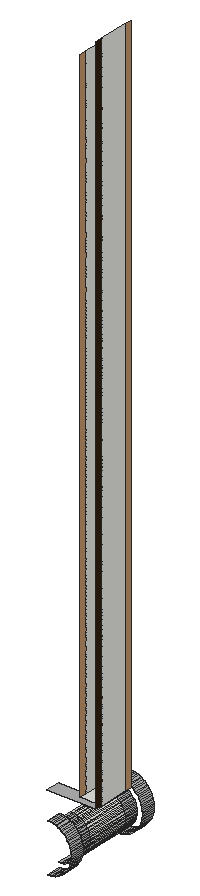
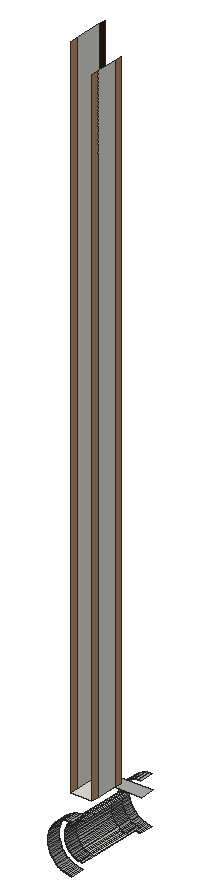
# SketchUp Ruby script. Lengths in inches.
U = 1.inch
M = Sketchup.active_model
def pt(a) = Geom::Point3d.new(a.map { |v| v * U })
def face(e, loops, mat)
  f = e.add_face(loops[0].map { |a| pt(a) })
  loops[1..].each { |l| e.add_face(l.map { |a| pt(a) }).erase! }
  f.material = f.back_material = mat if mat
  f
end
# faces: each face lists its corners as indices into pts; further lists are holes
def faces(e, pts, list, mat = nil) = list.each { |f| face(e, (f[0].is_a?(Array) ? f : [f]).map { |l| l.map { |i| pts[i] } }, mat) }
# xy, xz, yz: faces in a plane at the given z, y or x. An outline is a flat list of corners, or four numbers for a rectangle; further outlines are holes
def ring(l) = l.size == 4 ? [[l[0], l[1]], [l[2], l[1]], [l[2], l[3]], [l[0], l[3]]] : l.each_slice(2).to_a
def flat(e, list, mat, &to3) = list.each { |f| face(e, (f[0].is_a?(Array) ? f : [f]).map { |l| ring(l).map { |u, v| to3.(u, v) } }, mat) }
def xy(e, z, list, mat = nil) = flat(e, list, mat) { |x, y| [x, y, z] }
def xz(e, y, list, mat = nil) = flat(e, list, mat) { |x, z| [x, y, z] }
def yz(e, x, list, mat = nil) = flat(e, list, mat) { |y, z| [x, y, z] }
def lines(e, pts, list) = list.each { |a, b| e.add_line(pt(pts[a]), pt(pts[b])) }
# prism: a flat outline (further loops are holes) pulled along v
def prism(e, loops, v, mat = nil)
  f = face(e, loops, mat); d = Geom::Vector3d.new(v.map { |x| x * U })
  f.pushpull(f.normal.samedirection?(d) ? d.length : -d.length)
end
def box(e, o, s, mat = nil) = prism(e, [[o, [o[0] + s[0], o[1], o[2]], [o[0] + s[0], o[1] + s[1], o[2]], [o[0], o[1] + s[1], o[2]]]], [0, 0, s[2]], mat)
def at(x, y, z, deg = 0) = Geom::Transformation.translation(pt([x, y, z])) * Geom::Transformation.rotation(ORIGIN, Z_AXIS, deg.degrees)
def axes(o, x, y, z) = Geom::Transformation.new([*x, 0, *y, 0, *z, 0, *pt(o).to_a, 1])
def part(name) = M.definitions.add(name)
# library, detail: a bought-in or finely detailed component or shape, given as its bounding box
def library(name, o, s) = part(name).tap { |d| box(d.entities, o, s) }
def detail(e, o, s) = box(e.add_group.entities, o, s)
def put(e, d, t, mat = nil) = e.add_instance(d, t).tap { |i| i.material = mat if mat }
def group(e, t, mat = nil) = e.add_group.tap { |g| g.transformation = t; g.material = mat if mat }.entities
root = M.entities
M.materials.add("Panel-Opening1").color = [191, 148, 107]
M.materials.add("Stained Mahogany").color = [48, 33, 18]
M.materials.add("[Aluminum]").color = [178, 178, 178]
xy(root,65.29,[[211.71,132.28,211.79,133.02]],"[Aluminum]")
xy(root,65.33,[[211.71,127.79,211.79,128.53]],"[Aluminum]")
xy(root,65.58,[[211.71,129.28,211.78,131.53]])
xy(root,65.58,[[211.71,128.53,211.78,129.28],[211.71,131.53,211.78,132.28]],"[Aluminum]")
xy(root,67.55,[[211.71,129.28,211.78,131.53]])
xy(root,67.55,[[211.71,128.53,211.78,129.28],[211.71,131.53,211.78,132.28]],"[Aluminum]")
xy(root,67.8,[[211.71,127.79,211.79,128.53]],"[Aluminum]")
xy(root,67.84,[[211.71,132.28,211.79,133.02]],"[Aluminum]")
xy(root,68.11,[[211.84,129.66,212.96,131.53]])
xy(root,68.11,[[210.46,129.28,210.46,130.03,211.84,130.03,211.84,129.66,212.96,129.66,212.96,129.28]],"[Aluminum]")
yz(root,211.84,[[130.03,68.11,131.15,102.09]])
yz(root,211.84,[[129.66,68.11,130.03,102.09],[131.15,68.11,131.53,102.09]],"Panel-Opening1")
yz(root,212.67,[[129.28,66.4375,131.53,66.5],[129.28,66.5,131.53,66.5625],[129.28,66.5625,131.53,66.63],[129.28,66.63,131.53,66.69]])
yz(root,212.67,[[128.53,66.4375,129.28,66.5],[131.53,66.4375,132.28,66.5],[128.53,66.5,129.28,66.5625],[131.53,66.5,132.28,66.5625],[128.53,66.5625,129.28,66.63],
  [131.53,66.5625,132.28,66.63],[128.53,66.63,129.28,66.69],[131.53,66.63,132.28,66.69]],"[Aluminum]")
yz(root,212.92,[[127.79,66.48,128.53,66.57],[127.79,66.57,128.53,66.65]],"[Aluminum]")
yz(root,212.96,[[129.66,68.11,131.15,103.24]])
yz(root,212.96,[[131.15,68.11,131.53,103.24]],"Panel-Opening1")
yz(root,212.96,[[129.28,68.11,129.66,103.24]],"Stained Mahogany")
yz(root,212.96,[[132.28,66.48,133.02,66.5625],[132.28,66.5625,133.02,66.65]],"[Aluminum]")
p = [[211.79,128.53,65.33],[211.87,128.53,65.34],[211.87,127.79,65.34],[211.79,127.79,65.33],[211.95,128.53,65.35],[211.95,127.79,65.35],
  [211.875,132.28,65.3],[211.79,132.28,65.29],[211.79,133.02,65.29],[211.875,133.02,65.3],[211.96,132.28,65.31],[211.96,133.02,65.31],
  [212.04,132.28,65.33],[212.04,133.02,65.33],[212.11,132.28,65.35],[212.11,133.02,65.35],[212.03,128.53,65.37],[212.03,127.79,65.37],
  [212.1,128.53,65.39],[212.1,127.79,65.39],[212.17,128.53,65.42],[212.17,127.79,65.42],[212.25,128.53,65.46],[212.25,127.79,65.46],
  [212.19,132.28,65.38],[212.19,133.02,65.38],[212.26,132.28,65.42],[212.26,133.02,65.42],[212.34,132.28,65.46],[212.34,133.02,65.46],
  [212.32,128.53,65.5],[212.32,127.79,65.5],[212.38,128.53,65.54],[212.38,127.79,65.54],[212.45,128.53,65.58],[212.45,127.79,65.58],
  [212.41,132.28,65.5],[212.41,133.02,65.5],[212.47,132.28,65.55],[212.47,133.02,65.55],[212.54,132.28,65.6],[212.54,133.02,65.6],
  [212.51,128.53,65.64],[212.51,127.79,65.64],[212.57,128.53,65.69],[212.57,127.79,65.69],[211.84,129.28,65.59],[211.78,129.28,65.58],
  [211.78,128.53,65.58],[211.84,128.53,65.59],[211.9,129.28,65.6],[211.9,128.53,65.6],[211.96,129.28,65.61],[211.96,128.53,65.61],
  [212.02,129.28,65.63],[212.02,128.53,65.63],[212.08,129.28,65.66],[212.08,128.53,65.66],[211.78,131.53,65.58],[211.84,131.53,65.59],
  [211.9,131.53,65.6],[211.96,131.53,65.61],[212.02,131.53,65.63],[212.08,131.53,65.66],[211.78,132.28,65.58],[211.84,132.28,65.59],
  [211.9,132.28,65.6],[211.96,132.28,65.61],[212.02,132.28,65.63],[212.08,132.28,65.66],[212.6,132.28,65.66],[212.6,133.02,65.66],
  [212.62,128.53,65.75],[212.62,127.79,65.75],[212.14,129.28,65.68],[212.14,128.53,65.68],[212.19,129.28,65.71],[212.19,128.53,65.71],
  [212.25,129.28,65.75],[212.25,128.53,65.75],[212.3,129.28,65.78],[212.3,128.53,65.78],[212.14,131.53,65.68],[212.19,131.53,65.71],
  [212.25,131.53,65.75],[212.3,131.53,65.78],[212.14,132.28,65.68],[212.19,132.28,65.71],[212.25,132.28,65.75],[212.3,132.28,65.78],
  [212.65,132.28,65.72],[212.65,133.02,65.72],[212.7,132.28,65.79],[212.7,133.02,65.79],[212.67,128.53,65.8125],[212.67,127.79,65.8125],
  [212.72,128.53,65.88],[212.72,127.79,65.88],[212.35,129.28,65.82],[212.35,128.53,65.82],[212.39,129.28,65.87],[212.39,128.53,65.87],
  [212.35,131.53,65.82],[212.39,131.53,65.87],[212.35,132.28,65.82],[212.39,132.28,65.87],[212.75,132.28,65.85],[212.75,133.02,65.85],
  [212.76,128.53,65.95],[212.76,127.79,65.95],[212.79,128.53,66.02],[212.79,127.79,66.02],[212.44,129.28,65.92],[212.44,128.53,65.92],
  [212.48,129.28,65.97],[212.48,128.53,65.97],[212.44,131.53,65.92],[212.48,131.53,65.97],[212.44,132.28,65.92],[212.48,132.28,65.97],
  [212.79,132.28,65.93],[212.79,133.02,65.93],[212.83,132.28,66],[212.83,133.02,66],[212.83,128.53,66.09],[212.83,127.79,66.09],
  [212.51,129.28,66.02],[212.51,128.53,66.02],[212.55,129.28,66.07],[212.55,128.53,66.07],[212.51,131.53,66.02],[212.55,131.53,66.07],
  [212.51,132.28,66.02],[212.55,132.28,66.07],[212.87,132.28,66.08],[212.87,133.02,66.08],[212.85,128.53,66.17],[212.85,127.79,66.17],
  [212.57,129.28,66.13],[212.57,128.53,66.13],[212.6,129.28,66.1875],[212.6,128.53,66.1875],[212.57,131.53,66.13],[212.6,131.53,66.1875],
  [212.57,132.28,66.13],[212.6,132.28,66.1875],[212.89,132.28,66.15],[212.89,133.02,66.15],[212.875,128.53,66.25],[212.875,127.79,66.25],
  [212.89,128.53,66.32],[212.89,127.79,66.32],[212.625,129.28,66.25],[212.625,128.53,66.25],[212.64,129.28,66.31],[212.64,128.53,66.31],
  [212.625,131.53,66.25],[212.64,131.53,66.31],[212.625,132.28,66.25],[212.64,132.28,66.31],[212.92,132.28,66.23],[212.92,133.02,66.23],
  [212.9375,132.28,66.31],[212.9375,133.02,66.31],[212.91,128.53,66.4],[212.91,127.79,66.4],[212.66,129.28,66.37],[212.66,128.53,66.37],
  [212.66,131.53,66.37],[212.66,132.28,66.37],[212.95,132.28,66.4],[212.95,133.02,66.4],[212.92,128.53,66.48],[212.92,127.79,66.48],
  [212.67,129.28,66.4375],[212.67,128.53,66.4375],[212.67,131.53,66.4375],[212.67,132.28,66.4375],[212.96,132.28,66.48],[212.96,133.02,66.48],
  [212.92,128.53,66.65],[212.91,128.53,66.73],[212.91,127.79,66.73],[212.92,127.79,66.65],[212.95,132.28,66.73],[212.96,132.28,66.65],
  [212.96,133.02,66.65],[212.95,133.02,66.73],[212.89,128.53,66.81],[212.89,127.79,66.81],[212.66,129.28,66.76],[212.67,129.28,66.69],
  [212.67,128.53,66.69],[212.66,128.53,66.76],[212.67,131.53,66.69],[212.66,131.53,66.76],[212.67,132.28,66.69],[212.66,132.28,66.76],
  [212.9375,132.28,66.8125],[212.9375,133.02,66.8125],[212.875,128.53,66.88],[212.875,127.79,66.88],[212.625,129.28,66.88],[212.64,129.28,66.82],
  [212.64,128.53,66.82],[212.625,128.53,66.88],[212.64,131.53,66.82],[212.625,131.53,66.88],[212.64,132.28,66.82],[212.625,132.28,66.88],
  [212.92,132.28,66.9],[212.92,133.02,66.9],[212.85,128.53,66.96],[212.85,127.79,66.96],[212.57,129.28,67],[212.6,129.28,66.94],
  [212.6,128.53,66.94],[212.57,128.53,67],[212.6,131.53,66.94],[212.57,131.53,67],[212.6,132.28,66.94],[212.57,132.28,67],
  [212.89,132.28,66.98],[212.89,133.02,66.98],[212.83,128.53,67.04],[212.79,128.53,67.11],[212.79,127.79,67.11],[212.83,127.79,67.04],
  [212.55,129.28,67.06],[212.55,128.53,67.06],[212.55,131.53,67.06],[212.55,132.28,67.06],[212.87,132.28,67.05],[212.87,133.02,67.05],
  [212.76,128.53,67.18],[212.76,127.79,67.18],[212.48,129.28,67.16],[212.51,129.28,67.11],[212.51,128.53,67.11],[212.48,128.53,67.16],
  [212.51,131.53,67.11],[212.48,131.53,67.16],[212.51,132.28,67.11],[212.48,132.28,67.16],[212.79,132.28,67.2],[212.83,132.28,67.13],
  [212.83,133.02,67.13],[212.79,133.02,67.2],[212.71,128.53,67.25],[212.71,127.79,67.25],[212.39,129.28,67.26],[212.44,129.28,67.21],
  [212.44,128.53,67.21],[212.39,128.53,67.26],[212.44,131.53,67.21],[212.39,131.53,67.26],[212.44,132.28,67.21],[212.39,132.28,67.26],
  [212.75,132.28,67.27],[212.75,133.02,67.27],[212.67,128.53,67.32],[212.62,128.53,67.38],[212.62,127.79,67.38],[212.67,127.79,67.32],
  [212.25,129.28,67.38],[212.3,129.28,67.34],[212.3,128.53,67.34],[212.25,128.53,67.38],[212.35,129.28,67.3],[212.35,128.53,67.3],
  [212.3,131.53,67.34],[212.25,131.53,67.38],[212.35,131.53,67.3],[212.3,132.28,67.34],[212.25,132.28,67.38],[212.35,132.28,67.3],
  [212.65,132.28,67.41],[212.7,132.28,67.34],[212.7,133.02,67.34],[212.65,133.02,67.41],[212.5625,128.53,67.4375],[212.51,128.53,67.49],
  [212.51,127.79,67.49],[212.5625,127.79,67.4375],[212.08,129.28,67.47],[212.14,129.28,67.45],[212.14,128.53,67.45],[212.08,128.53,67.47],
  [212.19,129.28,67.42],[212.19,128.53,67.42],[212.14,131.53,67.45],[212.08,131.53,67.47],[212.19,131.53,67.42],[212.14,132.28,67.45],
  [212.08,132.28,67.47],[212.19,132.28,67.42],[212.59,132.28,67.47],[212.59,133.02,67.47],[212.45,128.53,67.54],[212.38,128.53,67.59],
  [212.38,127.79,67.59],[212.45,127.79,67.54],[211.78,129.28,67.55],[211.84,129.28,67.54],[211.84,128.53,67.54],[211.78,128.53,67.55],
  [211.9,129.28,67.53],[211.9,128.53,67.53],[211.96,129.28,67.51],[211.96,128.53,67.51],[212.02,129.28,67.5],[212.02,128.53,67.5],
  [211.84,131.53,67.54],[211.78,131.53,67.55],[211.9,131.53,67.53],[211.96,131.53,67.51],[212.02,131.53,67.5],[211.84,132.28,67.54],
  [211.78,132.28,67.55],[211.9,132.28,67.53],[211.96,132.28,67.51],[212.02,132.28,67.5],[212.47,132.28,67.58],[212.54,132.28,67.53],
  [212.54,133.02,67.53],[212.47,133.02,67.58],[212.3125,128.53,67.63],[212.24,128.53,67.67],[212.24,127.79,67.67],[212.3125,127.79,67.63],
  [212.34,132.28,67.67],[212.41,132.28,67.63],[212.41,133.02,67.63],[212.34,133.02,67.67],[212.1,128.53,67.73],[212.02,128.53,67.76],
  [212.02,127.79,67.76],[212.1,127.79,67.73],[212.17,128.53,67.71],[212.17,127.79,67.71],[212.11,132.28,67.78],[212.19,132.28,67.75],
  [212.19,133.02,67.75],[212.11,133.02,67.78],[212.26,132.28,67.71],[212.26,133.02,67.71],[211.87,128.53,67.79],[211.79,128.53,67.8],
  [211.79,127.79,67.8],[211.87,127.79,67.79],[211.95,128.53,67.78],[211.95,127.79,67.78],[211.79,132.28,67.84],[211.875,132.28,67.83],
  [211.875,133.02,67.83],[211.79,133.02,67.84],[211.96,132.28,67.82],[211.96,133.02,67.82],[212.04,132.28,67.8],[212.04,133.02,67.8]]
faces(root,p,[[0,1,2,3],[1,4,5,2],[6,7,8,9],[10,6,9,11],[12,10,11,13],[14,12,13,15],[4,16,17,5],[16,18,19,17],
  [18,20,21,19],[20,22,23,21],[24,14,15,25],[26,24,25,27],[28,26,27,29],[22,30,31,23],[30,32,33,31],[32,34,35,33],
  [36,28,29,37],[38,36,37,39],[40,38,39,41],[34,42,43,35],[42,44,45,43],[46,47,48,49],[50,46,49,51],[52,50,51,53],
  [54,52,53,55],[56,54,55,57],[59,58,64,65],[60,59,65,66],[61,60,66,67],[62,61,67,68],[63,62,68,69],[70,40,41,71],
  [44,72,73,45],[74,56,57,75],[76,74,75,77],[78,76,77,79],[80,78,79,81],[82,63,69,86],[83,82,86,87],[84,83,87,88],
  [85,84,88,89],[90,70,71,91],[92,90,91,93],[72,94,95,73],[94,96,97,95],[98,80,81,99],[100,98,99,101],[102,85,89,104],
  [103,102,104,105],[106,92,93,107],[96,108,109,97],[108,110,111,109],[112,100,101,113],[114,112,113,115],[116,103,105,118],[117,116,118,119],
  [120,106,107,121],[122,120,121,123],[110,124,125,111],[126,114,115,127],[128,126,127,129],[130,117,119,132],[131,130,132,133],[134,122,123,135],
  [124,136,137,125],[138,128,129,139],[140,138,139,141],[142,131,133,144],[143,142,144,145],[146,134,135,147],[136,148,149,137],[148,150,151,149],
  [152,140,141,153],[154,152,153,155],[156,143,145,158],[157,156,158,159],[160,146,147,161],[162,160,161,163],[150,164,165,151],[166,154,155,167],
  [168,157,159,169],[170,162,163,171],[164,172,173,165],[174,166,167,175],[176,168,169,177],[178,170,171,179],[180,181,182,183],[184,185,186,187],
  [181,188,189,182],[190,191,192,193],[195,194,196,197],[198,184,187,199],[188,200,201,189],[202,203,204,205],[203,190,193,204],[207,206,208,209],
  [206,195,197,208],[210,198,199,211],[200,212,213,201],[214,215,216,217],[215,202,205,216],[219,218,220,221],[218,207,209,220],[222,210,211,223],
  [224,225,226,227],[212,224,227,213],[228,214,217,229],[230,219,221,231],[232,222,223,233],[225,234,235,226],[236,237,238,239],[237,228,229,238],
  [241,240,242,243],[240,230,231,242],[244,245,246,247],[245,232,233,246],[234,248,249,235],[250,251,252,253],[251,236,239,252],[255,254,256,257],
  [254,241,243,256],[258,244,247,259],[260,261,262,263],[248,260,263,249],[264,265,266,267],[265,268,269,266],[268,250,253,269],[271,270,273,274],
  [270,272,275,273],[272,255,257,275],[276,277,278,279],[277,258,259,278],[280,281,282,283],[261,280,283,262],[284,285,286,287],[285,288,289,286],
  [288,264,267,289],[291,290,293,294],[290,292,295,293],[292,271,274,295],[296,276,279,297],[298,299,300,301],[281,298,301,282],[302,303,304,305],
  [303,306,307,304],[306,308,309,307],[308,310,311,309],[310,284,287,311],[313,312,317,318],[312,314,319,317],[314,315,320,319],[315,316,321,320],
  [316,291,294,321],[322,323,324,325],[323,296,297,324],[326,327,328,329],[299,326,329,300],[330,331,332,333],[331,322,325,332],[334,335,336,337],
  [338,334,337,339],[327,338,339,328],[340,341,342,343],[341,344,345,342],[344,330,333,345],[346,347,348,349],[350,346,349,351],[335,350,351,336],
  [352,353,354,355],[353,356,357,354],[356,358,359,357],[358,340,343,359]],"[Aluminum]")
faces(root,p,[[58,59,46,47],[59,60,50,46],[60,61,52,50],[61,62,54,52],[62,63,56,54],[63,82,74,56],[82,83,76,74],[83,84,78,76],
  [84,85,80,78],[85,102,98,80],[102,103,100,98],[103,116,112,100],[116,117,114,112],[117,130,126,114],[130,131,128,126],[131,142,138,128],
  [142,143,140,138],[143,156,152,140],[156,157,154,152],[157,168,166,154],[168,176,174,166],[194,195,190,191],[206,207,202,203],[195,206,203,190],
  [218,219,214,215],[207,218,215,202],[219,230,228,214],[240,241,236,237],[230,240,237,228],[254,255,250,251],[241,254,251,236],[270,271,264,265],
  [272,270,265,268],[255,272,268,250],[290,291,284,285],[292,290,285,288],[271,292,288,264],[312,313,302,303],[314,312,303,306],[315,314,306,308],
  [316,315,308,310],[291,316,310,284]])
